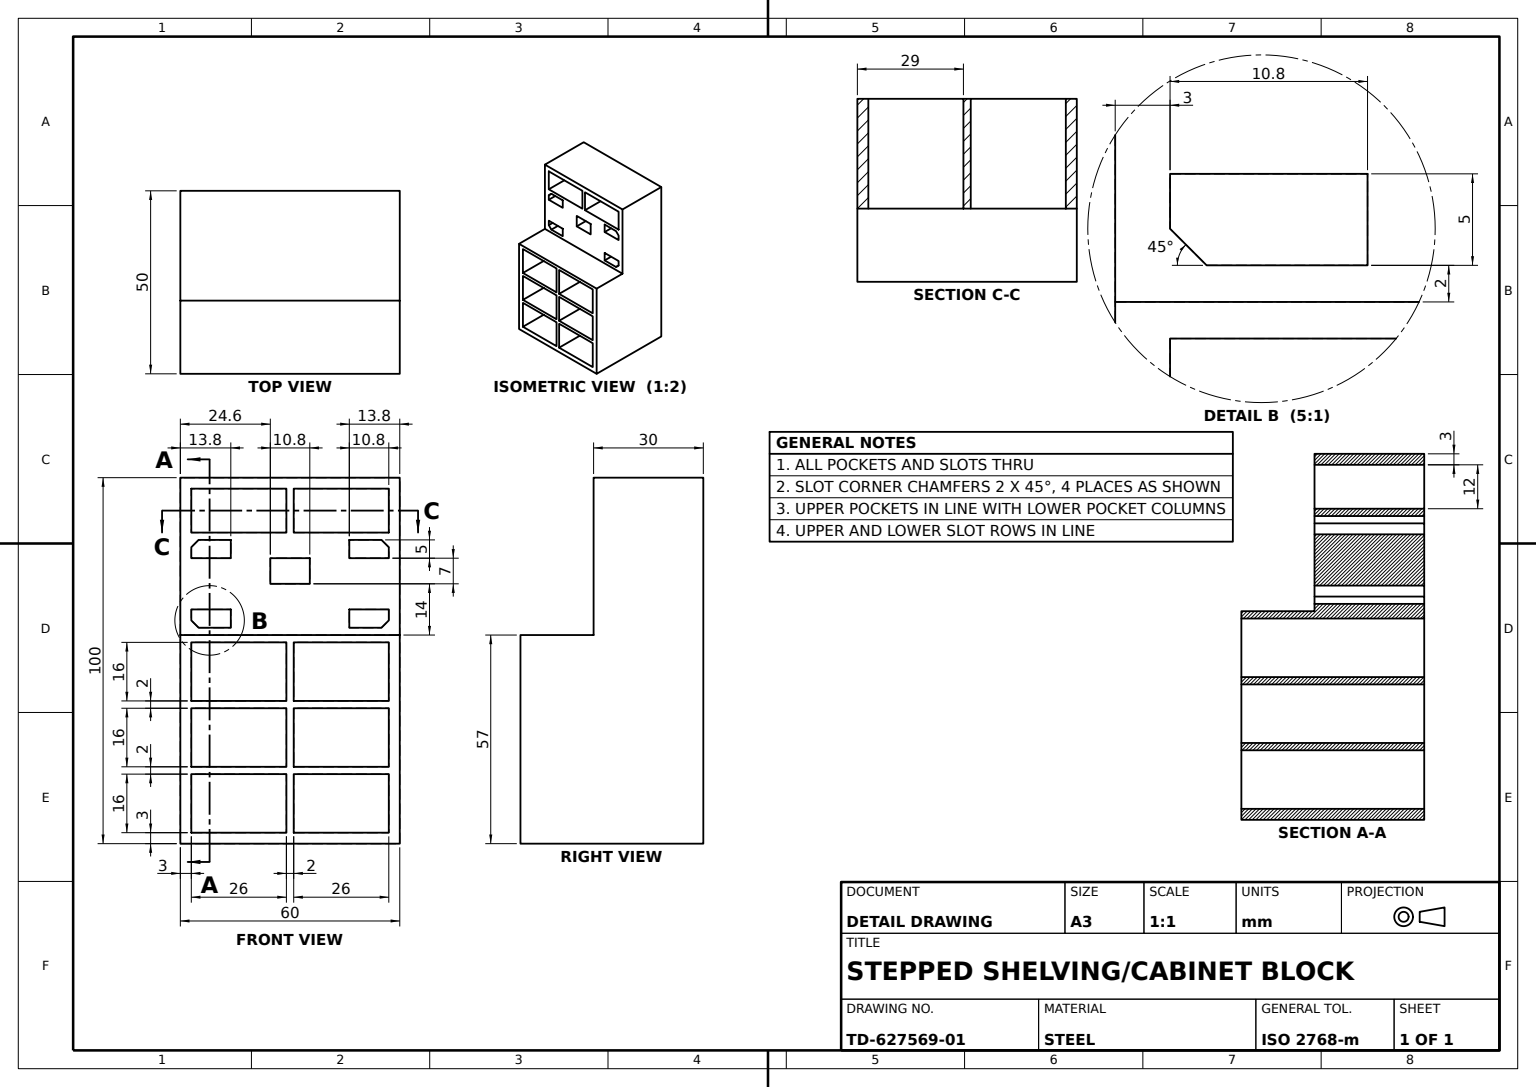
solid
v1 (27,35,30)
v2 (27,47,30)
e1 v1 v2 LINE
v3 (27,47,0)
e2 v3 v2 LINE
v4 (27,35,0)
e3 v4 v3 LINE
e4 v4 v1 LINE
face PLANE(AX(P(27,0,0),D(1,0,0),D(0,1,0))) rev [e1 -e2 -e3 e4]
v5 (-1,47,0)
v6 (-1,35,0)
e5 v5 v6 LINE
v7 (-27,47,0)
e6 v7 v5 LINE
v8 (-27,35,0)
e7 v7 v8 LINE
e8 v8 v6 LINE
v9 (-25,9,0)
v10 (-27,11,0)
e9 v9 v10 LINE
v11 (-16.2,9,0)
e10 v9 v11 LINE
v12 (-16.2,14,0)
e11 v12 v11 LINE
v13 (-27,14,0)
e12 v13 v12 LINE
e13 v13 v10 LINE
v14 (27,-31,0)
v15 (1,-31,0)
e14 v14 v15 LINE
v16 (1,-47,0)
e15 v15 v16 LINE
v17 (27,-47,0)
e16 v16 v17 LINE
e17 v17 v14 LINE
v18 (-1,-31,0)
v19 (-27,-31,0)
e18 v18 v19 LINE
v20 (-27,-47,0)
e19 v19 v20 LINE
v21 (-1,-47,0)
e20 v20 v21 LINE
e21 v21 v18 LINE
v22 (-16.2,33,0)
v23 (-16.2,28,0)
e22 v22 v23 LINE
v24 (-25,33,0)
e23 v24 v22 LINE
v25 (-27,31,0)
e24 v24 v25 LINE
v26 (-27,28,0)
e25 v25 v26 LINE
e26 v26 v23 LINE
v27 (-30,50,0)
v28 (-30,-50,0)
e27 v27 v28 LINE
v29 (30,50,0)
e28 v29 v27 LINE
v30 (30,-50,0)
e29 v30 v29 LINE
e30 v28 v30 LINE
v31 (-27,-29,0)
v32 (-1,-29,0)
e31 v31 v32 LINE
v33 (-1,-13,0)
e32 v32 v33 LINE
v34 (-27,-13,0)
e33 v33 v34 LINE
e34 v34 v31 LINE
v35 (-5.4,28,0)
v36 (5.4,28,0)
e35 v35 v36 LINE
v37 (-5.4,21,0)
e36 v35 v37 LINE
v38 (5.4,21,0)
e37 v37 v38 LINE
e38 v36 v38 LINE
v39 (16.2,33,0)
v40 (16.2,28,0)
e39 v39 v40 LINE
v41 (27,28,0)
e40 v40 v41 LINE
v42 (27,31,0)
e41 v42 v41 LINE
v43 (25,33,0)
e42 v43 v42 LINE
e43 v39 v43 LINE
v44 (27,-13,0)
v45 (1,-13,0)
e44 v44 v45 LINE
v46 (1,-29,0)
e45 v45 v46 LINE
v47 (27,-29,0)
e46 v46 v47 LINE
e47 v47 v44 LINE
v48 (1,47,0)
e48 v3 v48 LINE
v49 (1,35,0)
e49 v48 v49 LINE
e50 v49 v4 LINE
v50 (27,-11,0)
v51 (27,5,0)
e51 v50 v51 LINE
v52 (1,5,0)
e52 v51 v52 LINE
v53 (1,-11,0)
e53 v52 v53 LINE
e54 v53 v50 LINE
v54 (-1,-11,0)
v55 (-1,5,0)
e55 v54 v55 LINE
v56 (-27,5,0)
e56 v55 v56 LINE
v57 (-27,-11,0)
e57 v56 v57 LINE
e58 v57 v54 LINE
v58 (16.2,9,0)
v59 (25,9,0)
e59 v58 v59 LINE
v60 (27,11,0)
e60 v59 v60 LINE
v61 (27,14,0)
e61 v61 v60 LINE
v62 (16.2,14,0)
e62 v62 v61 LINE
e63 v62 v58 LINE
face PLANE(AX(P(0,0,0),D(0,0,-1),D(-1,0,0))) [-e5 -e6 e7 e8] [-e9 e10 -e11 -e12 e13] [e14 e15 e16 e17] [e18 e19 e20 e21] [-e22 -e23 e24 e25 e26] [-e27 -e28 -e29 -e30] [e31 e32 e33 e34] [-e35 e36 e37 -e38] [e39 e40 -e41 -e42 -e43] [e44 e45 e46 e47] [e48 e49 e50 e3] [e51 e52 e53 e54] [e55 e56 e57 e58] [e59 e60 -e61 -e62 e63]
v63 (-27,11,30)
e64 v10 v63 LINE
v64 (-27,14,30)
e65 v13 v64 LINE
e66 v64 v63 LINE
face PLANE(AX(P(-27,0,0),D(-1,0,0),D(0,-1,0))) rev [-e64 -e13 e65 e66]
v65 (27,-31,50)
v66 (1,-31,50)
e67 v65 v66 LINE
e68 v15 v66 LINE
e69 v14 v65 LINE
face PLANE(AX(P(1,-31,0),D(0,1,0),D(0,0,1))) rev [e67 -e68 -e14 e69]
v67 (1,47,30)
e70 v2 v67 LINE
e71 v48 v67 LINE
face PLANE(AX(P(0,47,0),D(0,1,0),D(-1,0,0))) rev [e2 e70 -e71 -e48]
v68 (16.2,33,30)
v69 (16.2,28,30)
e72 v68 v69 LINE
e73 v40 v69 LINE
e74 v39 v68 LINE
face PLANE(AX(P(16.2,0,0),D(-1,0,0),D(0,0,1))) rev [e72 -e73 -e39 e74]
v70 (-16.2,14,30)
e75 v12 v70 LINE
e76 v64 v70 LINE
face PLANE(AX(P(0,14,0),D(0,-1,0),D(0,0,-1))) [e12 e75 -e76 -e65]
v71 (-30,7,50)
v72 (-30,-50,50)
e77 v71 v72 LINE
v73 (-30,7,30)
e78 v71 v73 LINE
v74 (-30,50,30)
e79 v74 v73 LINE
e80 v74 v27 LINE
e81 v72 v28 LINE
face PLANE(AX(P(-30,-50,30),D(1,0,0),D(0,0,-1))) rev [-e77 e78 -e79 e80 e27 -e81]
v75 (27,5,50)
v76 (1,5,50)
e82 v75 v76 LINE
e83 v52 v76 LINE
e84 v51 v75 LINE
face PLANE(AX(P(1,5,0),D(0,1,0),D(0,0,1))) rev [e82 -e83 -e52 e84]
v77 (27,11,30)
e85 v60 v77 LINE
v78 (27,14,30)
e86 v78 v77 LINE
e87 v61 v78 LINE
face PLANE(AX(P(27,0,0),D(-1,0,0),D(0,-1,0))) [e61 e85 -e86 -e87]
v79 (-27,28,30)
e88 v26 v79 LINE
v80 (-16.2,28,30)
e89 v79 v80 LINE
e90 v23 v80 LINE
face PLANE(AX(P(0,28,0),D(0,-1,0),D(0,0,-1))) rev [e88 e89 -e90 -e26]
v81 (27,-47,50)
e91 v17 v81 LINE
e92 v81 v65 LINE
face PLANE(AX(P(27,-31,0),D(1,0,0),D(0,1,0))) rev [-e69 -e17 e91 e92]
v82 (-1,-11,50)
e93 v54 v82 LINE
v83 (-27,-11,50)
e94 v57 v83 LINE
e95 v83 v82 LINE
face PLANE(AX(P(-27,-11,0),D(0,-1,0),D(0,0,-1))) rev [-e93 -e58 e94 e95]
v84 (-1,-47,50)
e96 v21 v84 LINE
v85 (-1,-31,50)
e97 v84 v85 LINE
e98 v18 v85 LINE
face PLANE(AX(P(-1,-31,0),D(1,0,0),D(0,1,0))) rev [e96 e97 -e98 -e21]
v86 (30,-50,50)
e99 v72 v86 LINE
e100 v86 v30 LINE
face PLANE(AX(P(-30,-50,30),D(0,1,0),D(0,0,1))) rev [-e99 e81 e30 -e100]
v87 (1,-11,50)
e101 v53 v87 LINE
e102 v76 v87 LINE
face PLANE(AX(P(1,5,0),D(-1,0,0),D(0,-1,0))) rev [-e101 -e53 e83 e102]
v88 (27,-13,50)
e103 v44 v88 LINE
v89 (1,-13,50)
e104 v88 v89 LINE
e105 v45 v89 LINE
face PLANE(AX(P(1,-13,0),D(0,1,0),D(0,0,1))) rev [e103 e104 -e105 -e44]
v90 (30,7,30)
e106 v90 v73 LINE
v91 (30,7,50)
e107 v91 v71 LINE
e108 v91 v90 LINE
face PLANE(AX(P(-30,7,50),D(0,-1,0),D(0,0,-1))) rev [e106 -e78 -e107 e108]
v92 (16.2,14,30)
e109 v92 v78 LINE
e110 v62 v92 LINE
face PLANE(AX(P(0,14,0),D(0,-1,0),D(0,0,-1))) [e62 e87 -e109 -e110]
v93 (-27,47,30)
e111 v7 v93 LINE
v94 (-1,47,30)
e112 v5 v94 LINE
e113 v93 v94 LINE
face PLANE(AX(P(0,47,0),D(0,-1,0),D(0,0,-1))) [-e111 e6 e112 -e113]
v95 (-1,-13,50)
v96 (-27,-13,50)
e114 v95 v96 LINE
e115 v34 v96 LINE
e116 v33 v95 LINE
face PLANE(AX(P(-27,-13,0),D(0,1,0),D(0,0,1))) rev [e114 -e115 -e33 e116]
v97 (5.4,28,30)
e117 v36 v97 LINE
v98 (-5.4,28,30)
e118 v98 v97 LINE
e119 v35 v98 LINE
face PLANE(AX(P(0,28,0),D(0,-1,0),D(0,0,-1))) [e117 -e118 -e119 e35]
v99 (25,33,30)
e120 v43 v99 LINE
e121 v68 v99 LINE
face PLANE(AX(P(0,33,0),D(0,-1,0),D(0,0,-1))) [e43 e120 -e121 -e74]
v100 (27,31,30)
e122 v42 v100 LINE
e123 v99 v100 LINE
face PLANE(AX(P(29,29,0),D(-0.707106781,-0.707106781,0),D(0.707106781,-0.707106781,0))) [-e120 e42 e122 -e123]
v101 (27,28,30)
e124 v69 v101 LINE
e125 v41 v101 LINE
face PLANE(AX(P(0,28,0),D(0,-1,0),D(0,0,-1))) rev [-e40 e73 e124 -e125]
v102 (-16.2,9,30)
e126 v70 v102 LINE
e127 v11 v102 LINE
face PLANE(AX(P(-16.2,0,0),D(-1,0,0),D(0,0,1))) [-e126 -e75 e11 e127]
v103 (27,-11,50)
e128 v50 v103 LINE
e129 v103 v75 LINE
face PLANE(AX(P(27,5,0),D(1,0,0),D(0,1,0))) rev [-e84 -e51 e128 e129]
v104 (-25,9,30)
e130 v104 v63 LINE
e131 v9 v104 LINE
face PLANE(AX(P(-8,-8,0),D(0.707106781,0.707106781,0),D(-0.707106781,0.707106781,0))) [e64 -e130 -e131 e9]
v105 (1,-29,50)
e132 v46 v105 LINE
e133 v89 v105 LINE
face PLANE(AX(P(1,-13,0),D(-1,0,0),D(0,-1,0))) rev [-e132 -e45 e105 e133]
v106 (-5.4,21,30)
e134 v98 v106 LINE
e135 v37 v106 LINE
face PLANE(AX(P(-5.4,0,0),D(-1,0,0),D(0,0,1))) rev [e119 e134 -e135 -e36]
v107 (30,50,30)
e136 v107 v29 LINE
e137 v107 v74 LINE
face PLANE(AX(P(-30,50,30),D(0,-1,0),D(0,0,-1))) rev [e136 e28 -e80 -e137]
v108 (1,-47,50)
e138 v16 v108 LINE
e139 v108 v81 LINE
face PLANE(AX(P(1,-47,0),D(0,-1,0),D(0,0,-1))) rev [e138 e139 -e91 -e16]
e140 v86 v91 LINE
e141 v90 v107 LINE
face PLANE(AX(P(30,-50,30),D(-1,0,0),D(0,0,1))) rev [-e140 e100 e29 -e136 -e141 -e108]
v109 (-27,-29,50)
e142 v31 v109 LINE
v110 (-1,-29,50)
e143 v109 v110 LINE
e144 v32 v110 LINE
face PLANE(AX(P(-27,-29,0),D(0,-1,0),D(0,0,-1))) rev [e142 e143 -e144 -e31]
v111 (1,35,30)
e145 v111 v1 LINE
e146 v49 v111 LINE
face PLANE(AX(P(0,35,0),D(0,-1,0),D(1,0,0))) rev [e145 -e4 -e50 e146]
v112 (-1,5,50)
v113 (-27,5,50)
e147 v112 v113 LINE
e148 v56 v113 LINE
e149 v55 v112 LINE
face PLANE(AX(P(-27,5,0),D(0,1,0),D(0,0,1))) rev [e147 -e148 -e56 e149]
e150 v66 v108 LINE
face PLANE(AX(P(1,-31,0),D(-1,0,0),D(0,-1,0))) rev [-e15 e68 e150 -e138]
e151 v110 v95 LINE
face PLANE(AX(P(-1,-13,0),D(1,0,0),D(0,1,0))) rev [-e32 e144 e151 -e116]
v114 (-27,-31,50)
v115 (-27,-47,50)
e152 v114 v115 LINE
e153 v85 v114 LINE
e154 v115 v84 LINE
e155 v96 v109 LINE
e156 v87 v103 LINE
e157 v113 v83 LINE
e158 v82 v112 LINE
v116 (27,-29,50)
e159 v116 v88 LINE
e160 v105 v116 LINE
face PLANE(AX(P(0,0,50),D(0,0,-1),D(-1,0,0))) rev [-e67 -e92 -e139 -e150] [e140 e107 e77 e99] [-e152 -e153 -e97 -e154] [-e114 -e151 -e143 -e155] [-e102 -e82 -e129 -e156] [-e157 -e147 -e158 -e95] [-e104 -e159 -e160 -e133]
e161 v67 v111 LINE
face PLANE(AX(P(1,0,0),D(-1,0,0),D(0,-1,0))) rev [-e146 -e49 e71 e161]
v117 (-27,35,30)
e162 v93 v117 LINE
e163 v8 v117 LINE
face PLANE(AX(P(-27,0,0),D(-1,0,0),D(0,0,1))) rev [e162 -e163 -e7 e111]
face PLANE(AX(P(-1,5,0),D(1,0,0),D(0,1,0))) rev [e93 e158 -e149 -e55]
face PLANE(AX(P(-27,-13,0),D(-1,0,0),D(0,-1,0))) rev [-e34 e115 e155 -e142]
v118 (16.2,9,30)
e164 v92 v118 LINE
e165 v58 v118 LINE
face PLANE(AX(P(16.2,0,0),D(-1,0,0),D(0,0,1))) rev [e164 -e165 -e63 e110]
face PLANE(AX(P(-27,5,0),D(-1,0,0),D(0,-1,0))) rev [-e94 -e57 e148 e157]
v119 (-25,33,30)
v120 (-16.2,33,30)
e166 v119 v120 LINE
e167 v24 v119 LINE
e168 v22 v120 LINE
face PLANE(AX(P(0,33,0),D(0,-1,0),D(0,0,-1))) [-e166 -e167 e23 e168]
e169 v47 v116 LINE
face PLANE(AX(P(27,-13,0),D(1,0,0),D(0,1,0))) rev [e169 e159 -e103 -e47]
e170 v120 v80 LINE
face PLANE(AX(P(-16.2,0,0),D(-1,0,0),D(0,0,1))) [e22 e90 -e170 -e168]
e171 v19 v114 LINE
face PLANE(AX(P(-27,-31,0),D(0,1,0),D(0,0,1))) rev [e98 e153 -e171 -e18]
e172 v20 v115 LINE
face PLANE(AX(P(-27,-47,0),D(0,-1,0),D(0,0,-1))) rev [-e96 -e20 e172 e154]
v121 (25,9,30)
e173 v118 v121 LINE
e174 v59 v121 LINE
face PLANE(AX(P(0,9,0),D(0,-1,0),D(0,0,-1))) rev [-e59 e165 e173 -e174]
v122 (-1,35,30)
e175 v6 v122 LINE
e176 v94 v122 LINE
face PLANE(AX(P(-1,0,0),D(-1,0,0),D(0,0,1))) [-e112 e5 e175 -e176]
face PLANE(AX(P(-27,-31,0),D(-1,0,0),D(0,-1,0))) rev [e171 e152 -e172 -e19]
v123 (5.4,21,30)
e177 v106 v123 LINE
e178 v38 v123 LINE
face PLANE(AX(P(0,21,0),D(0,-1,0),D(0,0,-1))) rev [-e37 e135 e177 -e178]
e179 v121 v77 LINE
face PLANE(AX(P(8,-8,0),D(0.707106781,-0.707106781,0),D(0.707106781,0.707106781,0))) rev [e179 -e85 -e60 e174]
v124 (-27,31,30)
e180 v119 v124 LINE
e181 v25 v124 LINE
face PLANE(AX(P(-29,29,0),D(-0.707106781,0.707106781,0),D(-0.707106781,-0.707106781,0))) rev [e180 -e181 -e24 e167]
face PLANE(AX(P(1,-29,0),D(0,-1,0),D(0,0,-1))) rev [e132 e160 -e169 -e46]
e182 v117 v122 LINE
face PLANE(AX(P(0,35,0),D(0,-1,0),D(0,0,-1))) rev [-e8 e163 e182 -e175]
e183 v100 v101 LINE
face PLANE(AX(P(27,0,0),D(-1,0,0),D(0,-1,0))) [e41 e125 -e183 -e122]
e184 v97 v123 LINE
e185 v104 v102 LINE
e186 v124 v79 LINE
face PLANE(AX(P(0,0,30),D(0,0,-1),D(-1,0,0))) rev [e184 -e177 -e134 e118] [e126 -e185 e130 -e66 e76] [-e162 e113 e176 -e182] [e170 -e89 -e186 -e180 e166] [-e145 -e161 -e70 -e1] [-e124 -e72 e121 e123 e183] [e141 e137 e79 -e106] [e86 -e179 -e173 -e164 e109]
face PLANE(AX(P(5.4,0,0),D(-1,0,0),D(0,0,1))) [e178 -e184 -e117 e38]
face PLANE(AX(P(-27,0,0),D(-1,0,0),D(0,-1,0))) rev [e181 e186 -e88 -e25]
face PLANE(AX(P(1,-11,0),D(0,-1,0),D(0,0,-1))) rev [e156 -e128 -e54 e101]
face PLANE(AX(P(0,9,0),D(0,-1,0),D(0,0,-1))) rev [e131 e185 -e127 -e10]
